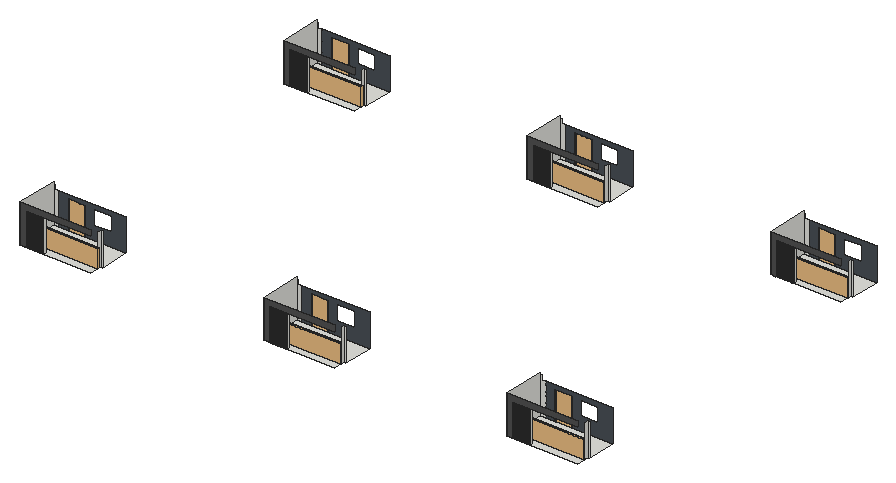
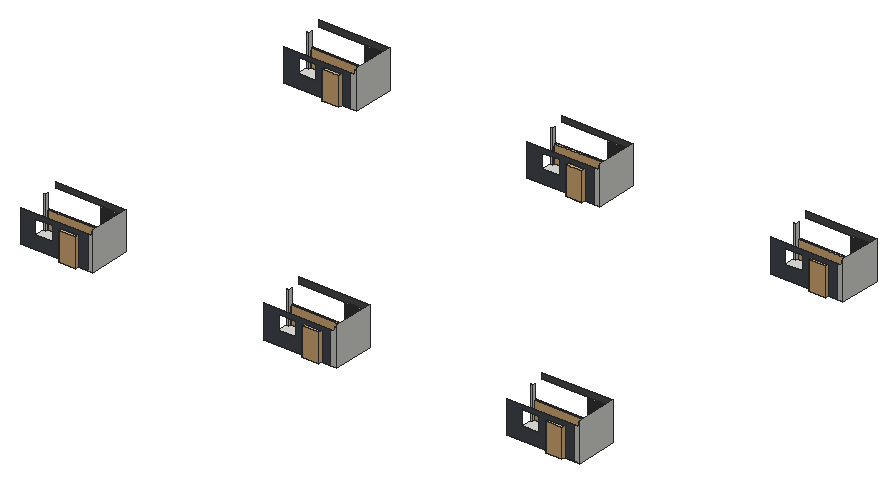
# SketchUp Ruby script. Lengths in inches.
U = 1.inch
M = Sketchup.active_model
def pt(a) = Geom::Point3d.new(a.map { |v| v * U })
def face(e, loops, mat)
  f = e.add_face(loops[0].map { |a| pt(a) })
  loops[1..].each { |l| e.add_face(l.map { |a| pt(a) }).erase! }
  f.material = f.back_material = mat if mat
  f
end
# faces: each face lists its corners as indices into pts; further lists are holes
def faces(e, pts, list, mat = nil) = list.each { |f| face(e, (f[0].is_a?(Array) ? f : [f]).map { |l| l.map { |i| pts[i] } }, mat) }
# xy, xz, yz: faces in a plane at the given z, y or x. An outline is a flat list of corners, or four numbers for a rectangle; further outlines are holes
def ring(l) = l.size == 4 ? [[l[0], l[1]], [l[2], l[1]], [l[2], l[3]], [l[0], l[3]]] : l.each_slice(2).to_a
def flat(e, list, mat, &to3) = list.each { |f| face(e, (f[0].is_a?(Array) ? f : [f]).map { |l| ring(l).map { |u, v| to3.(u, v) } }, mat) }
def xy(e, z, list, mat = nil) = flat(e, list, mat) { |x, y| [x, y, z] }
def xz(e, y, list, mat = nil) = flat(e, list, mat) { |x, z| [x, y, z] }
def yz(e, x, list, mat = nil) = flat(e, list, mat) { |y, z| [x, y, z] }
def lines(e, pts, list) = list.each { |a, b| e.add_line(pt(pts[a]), pt(pts[b])) }
# prism: a flat outline (further loops are holes) pulled along v
def prism(e, loops, v, mat = nil)
  f = face(e, loops, mat); d = Geom::Vector3d.new(v.map { |x| x * U })
  f.pushpull(f.normal.samedirection?(d) ? d.length : -d.length)
end
def box(e, o, s, mat = nil) = prism(e, [[o, [o[0] + s[0], o[1], o[2]], [o[0] + s[0], o[1] + s[1], o[2]], [o[0], o[1] + s[1], o[2]]]], [0, 0, s[2]], mat)
def at(x, y, z, deg = 0) = Geom::Transformation.translation(pt([x, y, z])) * Geom::Transformation.rotation(ORIGIN, Z_AXIS, deg.degrees)
def axes(o, x, y, z) = Geom::Transformation.new([*x, 0, *y, 0, *z, 0, *pt(o).to_a, 1])
def part(name) = M.definitions.add(name)
# library, detail: a bought-in or finely detailed component or shape, given as its bounding box
def library(name, o, s) = part(name).tap { |d| box(d.entities, o, s) }
def detail(e, o, s) = box(e.add_group.entities, o, s)
def put(e, d, t, mat = nil) = e.add_instance(d, t).tap { |i| i.material = mat if mat }
def group(e, t, mat = nil) = e.add_group.tap { |g| g.transformation = t; g.material = mat if mat }.entities
root = M.entities
M.materials.add("[0030_OldLace]").color = [86, 53, 24]
M.materials.add("[0135_DarkGray]").color = [81, 81, 81]
M.materials.add("[Formica Blue]").color = [73, 80, 86]
c1 = library("Glass Railing",[0,0,0],[139.5,4.76,42])
c2 = library("door (1)",[38.93,25.48,0],[40,9.94,82.68])
xy(root,143.875,[[[137.5,412.04,348.1875,412.04,348.1875,447.84,353.97,447.84,353.97,535.375,231.3,535.375,231.3,540.48,183.3,540.48,183.3,535.375,137.5,535.375],[175.88,414.01,179.51,418.7],[154.69,414.01,158.32,418.7],[160.01,414.01,163.63,418.7],[165.19,414.01,168.82,418.7],[170.38,414.01,174.01,418.7],[181.38,414.01,185.01,418.7],[186.88,414.01,190.51,418.7],[192.38,414.01,196.01,418.7],[197.88,414.01,201.51,418.7],[203.38,414.01,207.01,418.7]],[[861.9375,412.04,1072.625,412.04,1072.625,447.84,1078.41,447.84,1078.41,535.375,955.74,535.375,955.74,540.48,907.74,540.48,907.74,535.375,861.9375,535.375],[879.13,414.01,882.76,418.7],[884.44,414.01,888.07,418.7],[889.63,414.01,893.26,418.7],[894.82,414.01,898.44,418.7],[900.32,414.01,903.94,418.7],[905.82,414.01,909.44,418.7],[911.32,414.01,914.94,418.7],[916.82,414.01,920.44,418.7],[922.32,414.01,925.94,418.7],[927.82,414.01,931.44,418.7]],[[1586.375,412.04,1797.0625,412.04,1797.0625,447.84,1802.84,447.84,1802.84,535.375,1680.17,535.375,1680.17,540.48,1632.17,540.48,1632.17,535.375,1586.375,535.375],[1624.76,414.01,1628.38,418.7],[1603.57,414.01,1607.19,418.7],[1608.88,414.01,1612.51,418.7],[1614.07,414.01,1617.69,418.7],[1619.26,414.01,1622.88,418.7],[1630.26,414.01,1633.88,418.7],[1635.76,414.01,1639.38,418.7],[1641.26,414.01,1644.88,418.7],[1646.76,414.01,1650.38,418.7],[1652.26,414.01,1655.88,418.7]],[[137.5,1392.39,348.1875,1392.39,348.1875,1428.19,353.97,1428.19,353.97,1515.73,231.3,1515.73,231.3,1520.83,183.3,1520.83,183.3,1515.73,137.5,1515.73],[175.88,1394.36,179.51,1399.05],[154.69,1394.36,158.32,1399.05],[160.01,1394.36,163.63,1399.05],[165.19,1394.36,168.82,1399.05],[170.38,1394.36,174.01,1399.05],[181.38,1394.36,185.01,1399.05],[186.88,1394.36,190.51,1399.05],[192.38,1394.36,196.01,1399.05],[197.88,1394.36,201.51,1399.05],[203.38,1394.36,207.01,1399.05]],[[861.9375,1392.39,1072.625,1392.39,1072.625,1428.19,1078.41,1428.19,1078.41,1515.73,955.74,1515.73,955.74,1520.83,907.74,1520.83,907.74,1515.73,861.9375,1515.73],[879.13,1394.36,882.76,1399.05],[884.44,1394.36,888.07,1399.05],[889.63,1394.36,893.26,1399.05],[894.82,1394.36,898.44,1399.05],[900.32,1394.36,903.94,1399.05],[905.82,1394.36,909.44,1399.05],[911.32,1394.36,914.94,1399.05],[916.82,1394.36,920.44,1399.05],[922.32,1394.36,925.94,1399.05],[927.82,1394.36,931.44,1399.05]],
  [[1586.375,1392.39,1797.0625,1392.39,1797.0625,1428.19,1802.84,1428.19,1802.84,1515.73,1680.17,1515.73,1680.17,1520.83,1632.17,1520.83,1632.17,1515.73,1586.375,1515.73],[1624.76,1394.36,1628.38,1399.05],[1603.57,1394.36,1607.19,1399.05],[1608.88,1394.36,1612.51,1399.05],[1614.07,1394.36,1617.69,1399.05],[1619.26,1394.36,1622.88,1399.05],[1630.26,1394.36,1633.88,1399.05],[1635.76,1394.36,1639.38,1399.05],[1641.26,1394.36,1644.88,1399.05],[1646.76,1394.36,1650.38,1399.05],[1652.26,1394.36,1655.88,1399.05]]])
xz(root,412.04,[[137.5,143.875,153.26,143.875,153.26,240.625,348.1875,240.625,348.1875,258.25,137.5,258.25],[861.9375,143.875,877.69,143.875,877.69,240.625,1072.625,240.625,1072.625,258.25,861.9375,258.25],[1586.375,143.875,1602.13,143.875,1602.13,240.625,1797.0625,240.625,1797.0625,258.25,1586.375,258.25]],"[0135_DarkGray]")
xz(root,414.01,[[154.69,143.875,158.32,240.625],[160.01,143.875,163.63,240.625],[165.19,143.875,168.82,240.625],[170.38,143.875,174.01,240.625],[175.88,143.875,179.51,240.625],
  [181.38,143.875,185.01,240.625],[186.88,143.875,190.51,240.625],[192.38,143.875,196.01,240.625],[197.88,143.875,201.51,240.625],[203.38,143.875,207.01,240.625],
  [1603.57,143.875,1607.19,240.625],[1608.88,143.875,1612.51,240.625],[1614.07,143.875,1617.69,240.625],[1619.26,143.875,1622.88,240.625],[1624.76,143.875,1628.38,240.625],
  [1630.26,143.875,1633.88,240.625],[1635.76,143.875,1639.38,240.625],[1641.26,143.875,1644.88,240.625],[1646.76,143.875,1650.38,240.625],[1652.26,143.875,1655.88,240.625]])
xz(root,414.01,[[879.13,143.875,882.76,240.625],[884.44,143.875,888.07,240.625],[889.63,143.875,893.26,240.625],[894.82,143.875,898.44,240.625],[900.32,143.875,903.94,240.625],
  [905.82,143.875,909.44,240.625],[911.32,143.875,914.94,240.625],[916.82,143.875,920.44,240.625],[922.32,143.875,925.94,240.625],[927.82,143.875,931.44,240.625]],"[0030_OldLace]")
xz(root,418.7,[[154.69,143.875,158.32,240.625],[160.01,143.875,163.63,240.625],[165.19,143.875,168.82,240.625],[170.38,143.875,174.01,240.625],[175.88,143.875,179.51,240.625],
  [181.38,143.875,185.01,240.625],[186.88,143.875,190.51,240.625],[192.38,143.875,196.01,240.625],[197.88,143.875,201.51,240.625],[203.38,143.875,207.01,240.625],
  [879.13,143.875,882.76,240.625],[884.44,143.875,888.07,240.625],[889.63,143.875,893.26,240.625],[894.82,143.875,898.44,240.625],[900.32,143.875,903.94,240.625],
  [905.82,143.875,909.44,240.625],[911.32,143.875,914.94,240.625],[916.82,143.875,920.44,240.625],[922.32,143.875,925.94,240.625],[927.82,143.875,931.44,240.625],
  [1603.57,143.875,1607.19,240.625],[1608.88,143.875,1612.51,240.625],[1614.07,143.875,1617.69,240.625],[1619.26,143.875,1622.88,240.625],[1624.76,143.875,1628.38,240.625],
  [1630.26,143.875,1633.88,240.625],[1635.76,143.875,1639.38,240.625],[1641.26,143.875,1644.88,240.625],[1646.76,143.875,1650.38,240.625],[1652.26,143.875,1655.88,240.625]])
xz(root,447.84,[[348.1875,143.875,353.97,240.625],[1072.625,143.875,1078.41,240.625],[1797.0625,143.875,1802.84,240.625]])
xz(root,535.375,[[137.5,143.875,153.26,143.875,153.26,240.625,141.63,240.625,141.63,252.25,137.5,252.25],[861.9375,143.875,877.69,143.875,877.69,240.625,866.07,240.625,866.07,252.25,861.9375,252.25],[1586.375,143.875,1602.13,143.875,1602.13,240.625,1590.51,240.625,1590.51,252.25,1586.375,252.25]])
xz(root,535.375,[[[153.26,143.875,183.3,143.875,183.3,227.875,231.3,227.875,231.3,143.875,353.97,143.875,353.97,240.625,153.26,240.625],[258.09,183.6875,309.84,227.875]],[[877.69,143.875,907.74,143.875,907.74,227.875,955.74,227.875,955.74,143.875,1078.41,143.875,1078.41,240.625,877.69,240.625],[982.53,183.6875,1034.28,227.875]],[[1602.13,143.875,1632.17,143.875,1632.17,227.875,1680.17,227.875,1680.17,143.875,1802.84,143.875,1802.84,240.625,1602.13,240.625],[1706.96,183.6875,1758.71,227.875]]],"[Formica Blue]")
xz(root,1392.39,[[137.5,143.875,153.26,143.875,153.26,240.625,348.1875,240.625,348.1875,258.25,137.5,258.25],[861.9375,143.875,877.69,143.875,877.69,240.625,1072.625,240.625,1072.625,258.25,861.9375,258.25],[1586.375,143.875,1602.13,143.875,1602.13,240.625,1797.0625,240.625,1797.0625,258.25,1586.375,258.25]],"[0135_DarkGray]")
xz(root,1394.36,[[154.69,143.875,158.32,240.625],[160.01,143.875,163.63,240.625],[165.19,143.875,168.82,240.625],[170.38,143.875,174.01,240.625],[175.88,143.875,179.51,240.625],
  [181.38,143.875,185.01,240.625],[186.88,143.875,190.51,240.625],[192.38,143.875,196.01,240.625],[197.88,143.875,201.51,240.625],[203.38,143.875,207.01,240.625],
  [879.13,143.875,882.76,240.625],[884.44,143.875,888.07,240.625],[889.63,143.875,893.26,240.625],[894.82,143.875,898.44,240.625],[900.32,143.875,903.94,240.625],
  [905.82,143.875,909.44,240.625],[911.32,143.875,914.94,240.625],[916.82,143.875,920.44,240.625],[922.32,143.875,925.94,240.625],[927.82,143.875,931.44,240.625],
  [1603.57,143.875,1607.19,240.625],[1608.88,143.875,1612.51,240.625],[1614.07,143.875,1617.69,240.625],[1619.26,143.875,1622.88,240.625],[1624.76,143.875,1628.38,240.625],
  [1630.26,143.875,1633.88,240.625],[1635.76,143.875,1639.38,240.625],[1641.26,143.875,1644.88,240.625],[1646.76,143.875,1650.38,240.625],[1652.26,143.875,1655.88,240.625]])
xz(root,1399.05,[[154.69,143.875,158.32,240.625],[160.01,143.875,163.63,240.625],[165.19,143.875,168.82,240.625],[170.38,143.875,174.01,240.625],[175.88,143.875,179.51,240.625],
  [181.38,143.875,185.01,240.625],[186.88,143.875,190.51,240.625],[192.38,143.875,196.01,240.625],[197.88,143.875,201.51,240.625],[203.38,143.875,207.01,240.625],
  [879.13,143.875,882.76,240.625],[884.44,143.875,888.07,240.625],[889.63,143.875,893.26,240.625],[894.82,143.875,898.44,240.625],[900.32,143.875,903.94,240.625],
  [905.82,143.875,909.44,240.625],[911.32,143.875,914.94,240.625],[916.82,143.875,920.44,240.625],[922.32,143.875,925.94,240.625],[927.82,143.875,931.44,240.625],
  [1603.57,143.875,1607.19,240.625],[1608.88,143.875,1612.51,240.625],[1614.07,143.875,1617.69,240.625],[1619.26,143.875,1622.88,240.625],[1624.76,143.875,1628.38,240.625],
  [1630.26,143.875,1633.88,240.625],[1635.76,143.875,1639.38,240.625],[1641.26,143.875,1644.88,240.625],[1646.76,143.875,1650.38,240.625],[1652.26,143.875,1655.88,240.625]])
xz(root,1428.19,[[348.1875,143.875,353.97,240.625],[1072.625,143.875,1078.41,240.625],[1797.0625,143.875,1802.84,240.625]])
xz(root,1515.73,[[137.5,143.875,153.26,143.875,153.26,240.625,141.63,240.625,141.63,252.25,137.5,252.25],[861.9375,143.875,877.69,143.875,877.69,240.625,866.07,240.625,866.07,252.25,861.9375,252.25],[1586.375,143.875,1602.13,143.875,1602.13,240.625,1590.51,240.625,1590.51,252.25,1586.375,252.25]])
xz(root,1515.73,[[[153.26,143.875,183.3,143.875,183.3,227.875,231.3,227.875,231.3,143.875,353.97,143.875,353.97,240.625,153.26,240.625],[258.09,183.6875,309.84,227.875]],[[877.69,143.875,907.74,143.875,907.74,227.875,955.74,227.875,955.74,143.875,1078.41,143.875,1078.41,240.625,877.69,240.625],[982.53,183.6875,1034.28,227.875]],[[1602.13,143.875,1632.17,143.875,1632.17,227.875,1680.17,227.875,1680.17,143.875,1802.84,143.875,1802.84,240.625,1602.13,240.625],[1706.96,183.6875,1758.71,227.875]]],"[Formica Blue]")
yz(root,137.5,[[412.04,143.875,535.375,258.25],[1392.39,143.875,1515.73,258.25]])
yz(root,154.69,[[414.01,143.875,418.7,240.625],[1394.36,143.875,1399.05,240.625]])
yz(root,158.32,[[414.01,143.875,418.7,240.625],[1394.36,143.875,1399.05,240.625]])
yz(root,160.01,[[414.01,143.875,418.7,240.625],[1394.36,143.875,1399.05,240.625]])
yz(root,163.63,[[414.01,143.875,418.7,240.625],[1394.36,143.875,1399.05,240.625]])
yz(root,165.19,[[414.01,143.875,418.7,240.625],[1394.36,143.875,1399.05,240.625]])
yz(root,168.82,[[414.01,143.875,418.7,240.625],[1394.36,143.875,1399.05,240.625]])
yz(root,170.38,[[414.01,143.875,418.7,240.625],[1394.36,143.875,1399.05,240.625]])
yz(root,174.01,[[414.01,143.875,418.7,240.625],[1394.36,143.875,1399.05,240.625]])
yz(root,175.88,[[414.01,143.875,418.7,240.625],[1394.36,143.875,1399.05,240.625]])
yz(root,179.51,[[414.01,143.875,418.7,240.625],[1394.36,143.875,1399.05,240.625]])
yz(root,181.38,[[414.01,143.875,418.7,240.625],[1394.36,143.875,1399.05,240.625]])
yz(root,183.3,[[535.375,143.875,540.48,227.875],[1515.73,143.875,1520.83,227.875]])
yz(root,185.01,[[414.01,143.875,418.7,240.625],[1394.36,143.875,1399.05,240.625]])
yz(root,186.88,[[414.01,143.875,418.7,240.625],[1394.36,143.875,1399.05,240.625]])
yz(root,190.51,[[414.01,143.875,418.7,240.625],[1394.36,143.875,1399.05,240.625]])
yz(root,192.38,[[414.01,143.875,418.7,240.625],[1394.36,143.875,1399.05,240.625]])
yz(root,196.01,[[414.01,143.875,418.7,240.625],[1394.36,143.875,1399.05,240.625]])
yz(root,197.88,[[414.01,143.875,418.7,240.625],[1394.36,143.875,1399.05,240.625]])
yz(root,201.51,[[414.01,143.875,418.7,240.625],[1394.36,143.875,1399.05,240.625]])
yz(root,203.38,[[414.01,143.875,418.7,240.625],[1394.36,143.875,1399.05,240.625]])
yz(root,207.01,[[414.01,143.875,418.7,240.625],[1394.36,143.875,1399.05,240.625]])
yz(root,231.3,[[535.375,143.875,540.48,227.875],[1515.73,143.875,1520.83,227.875]])
yz(root,348.1875,[[438.72,143.875,438.72,174.69,441.04,174.69,441.04,176.39,438.72,176.39,438.72,240.625,447.84,240.625,447.84,143.875],[1419.07,143.875,1419.07,174.69,1421.39,174.69,1421.39,176.39,1419.07,176.39,1419.07,240.625,1428.19,240.625,1428.19,143.875]])
yz(root,861.9375,[[412.04,143.875,535.375,258.25],[1392.39,143.875,1515.73,258.25]])
yz(root,879.13,[[414.01,143.875,418.7,240.625],[1394.36,143.875,1399.05,240.625]])
yz(root,882.76,[[414.01,143.875,418.7,240.625],[1394.36,143.875,1399.05,240.625]])
yz(root,884.44,[[414.01,143.875,418.7,240.625],[1394.36,143.875,1399.05,240.625]])
yz(root,888.07,[[414.01,143.875,418.7,240.625],[1394.36,143.875,1399.05,240.625]])
yz(root,889.63,[[414.01,143.875,418.7,240.625],[1394.36,143.875,1399.05,240.625]])
yz(root,893.26,[[414.01,143.875,418.7,240.625],[1394.36,143.875,1399.05,240.625]])
yz(root,894.82,[[414.01,143.875,418.7,240.625],[1394.36,143.875,1399.05,240.625]])
yz(root,898.44,[[414.01,143.875,418.7,240.625],[1394.36,143.875,1399.05,240.625]])
yz(root,900.32,[[414.01,143.875,418.7,240.625],[1394.36,143.875,1399.05,240.625]])
yz(root,903.94,[[414.01,143.875,418.7,240.625],[1394.36,143.875,1399.05,240.625]])
yz(root,905.82,[[414.01,143.875,418.7,240.625],[1394.36,143.875,1399.05,240.625]])
yz(root,907.74,[[535.375,143.875,540.48,227.875],[1515.73,143.875,1520.83,227.875]])
yz(root,909.44,[[414.01,143.875,418.7,240.625],[1394.36,143.875,1399.05,240.625]])
yz(root,911.32,[[414.01,143.875,418.7,240.625],[1394.36,143.875,1399.05,240.625]])
yz(root,914.94,[[414.01,143.875,418.7,240.625],[1394.36,143.875,1399.05,240.625]])
yz(root,916.82,[[414.01,143.875,418.7,240.625],[1394.36,143.875,1399.05,240.625]])
yz(root,920.44,[[414.01,143.875,418.7,240.625],[1394.36,143.875,1399.05,240.625]])
yz(root,922.32,[[414.01,143.875,418.7,240.625],[1394.36,143.875,1399.05,240.625]])
yz(root,925.94,[[414.01,143.875,418.7,240.625],[1394.36,143.875,1399.05,240.625]])
yz(root,927.82,[[414.01,143.875,418.7,240.625],[1394.36,143.875,1399.05,240.625]])
yz(root,931.44,[[414.01,143.875,418.7,240.625],[1394.36,143.875,1399.05,240.625]])
yz(root,955.74,[[535.375,143.875,540.48,227.875],[1515.73,143.875,1520.83,227.875]])
yz(root,1072.625,[[438.72,143.875,438.72,174.69,441.04,174.69,441.04,176.39,438.72,176.39,438.72,240.625,447.84,240.625,447.84,143.875],[1419.07,143.875,1419.07,174.69,1421.39,174.69,1421.39,176.39,1419.07,176.39,1419.07,240.625,1428.19,240.625,1428.19,143.875]])
yz(root,1586.375,[[412.04,143.875,535.375,258.25],[1392.39,143.875,1515.73,258.25]])
yz(root,1603.57,[[414.01,143.875,418.7,240.625],[1394.36,143.875,1399.05,240.625]])
yz(root,1607.19,[[414.01,143.875,418.7,240.625],[1394.36,143.875,1399.05,240.625]])
yz(root,1608.88,[[414.01,143.875,418.7,240.625],[1394.36,143.875,1399.05,240.625]])
yz(root,1612.51,[[414.01,143.875,418.7,240.625],[1394.36,143.875,1399.05,240.625]])
yz(root,1614.07,[[414.01,143.875,418.7,240.625],[1394.36,143.875,1399.05,240.625]])
yz(root,1617.69,[[414.01,143.875,418.7,240.625],[1394.36,143.875,1399.05,240.625]])
yz(root,1619.26,[[414.01,143.875,418.7,240.625],[1394.36,143.875,1399.05,240.625]])
yz(root,1622.88,[[414.01,143.875,418.7,240.625],[1394.36,143.875,1399.05,240.625]])
yz(root,1624.76,[[414.01,143.875,418.7,240.625],[1394.36,143.875,1399.05,240.625]])
yz(root,1628.38,[[414.01,143.875,418.7,240.625],[1394.36,143.875,1399.05,240.625]])
yz(root,1630.26,[[414.01,143.875,418.7,240.625],[1394.36,143.875,1399.05,240.625]])
yz(root,1632.17,[[535.375,143.875,540.48,227.875],[1515.73,143.875,1520.83,227.875]])
yz(root,1633.88,[[414.01,143.875,418.7,240.625],[1394.36,143.875,1399.05,240.625]])
yz(root,1635.76,[[414.01,143.875,418.7,240.625],[1394.36,143.875,1399.05,240.625]])
yz(root,1639.38,[[414.01,143.875,418.7,240.625],[1394.36,143.875,1399.05,240.625]])
yz(root,1641.26,[[414.01,143.875,418.7,240.625],[1394.36,143.875,1399.05,240.625]])
yz(root,1644.88,[[414.01,143.875,418.7,240.625],[1394.36,143.875,1399.05,240.625]])
yz(root,1646.76,[[414.01,143.875,418.7,240.625],[1394.36,143.875,1399.05,240.625]])
yz(root,1650.38,[[414.01,143.875,418.7,240.625],[1394.36,143.875,1399.05,240.625]])
yz(root,1652.26,[[414.01,143.875,418.7,240.625],[1394.36,143.875,1399.05,240.625]])
yz(root,1655.88,[[414.01,143.875,418.7,240.625],[1394.36,143.875,1399.05,240.625]])
yz(root,1680.17,[[535.375,143.875,540.48,227.875],[1515.73,143.875,1520.83,227.875]])
yz(root,1797.0625,[[438.72,143.875,438.72,174.69,441.04,174.69,441.04,176.39,438.72,176.39,438.72,240.625,447.84,240.625,447.84,143.875],[1419.07,143.875,1419.07,174.69,1421.39,174.69,1421.39,176.39,1419.07,176.39,1419.07,240.625,1428.19,240.625,1428.19,143.875]])
put(root,c1,axes([1625.73,1416.01,143.84],[1.22818,0,0],[0,1.27,0],[0,0,1.27]))
put(root,c1,axes([901.29,1416.01,143.84],[1.22818,0,0],[0,1.27,0],[0,0,1.27]))
put(root,c1,axes([176.86,1416.01,143.84],[1.22818,0,0],[0,1.27,0],[0,0,1.27]))
put(root,c1,axes([901.29,435.66,143.84],[1.22818,0,0],[0,1.27,0],[0,0,1.27]))
put(root,c1,axes([1625.73,435.66,143.84],[1.22818,0,0],[0,1.27,0],[0,0,1.27]))
put(root,c1,axes([176.86,435.66,143.84],[1.22818,0,0],[0,1.27,0],[0,0,1.27]))
put(root,c2,axes([1582.69,1490.24,143.875],[1.2351,0,0],[0,1,0],[0,0,1.016]))
put(root,c2,axes([858.25,1490.24,143.875],[1.2351,0,0],[0,1,0],[0,0,1.016]))
put(root,c2,axes([133.81,1490.24,143.875],[1.2351,0,0],[0,1,0],[0,0,1.016]))
put(root,c2,axes([858.25,509.89,143.875],[1.2351,0,0],[0,1,0],[0,0,1.016]))
put(root,c2,axes([1582.69,509.89,143.875],[1.2351,0,0],[0,1,0],[0,0,1.016]))
put(root,c2,axes([133.81,509.89,143.875],[1.2351,0,0],[0,1,0],[0,0,1.016]))
